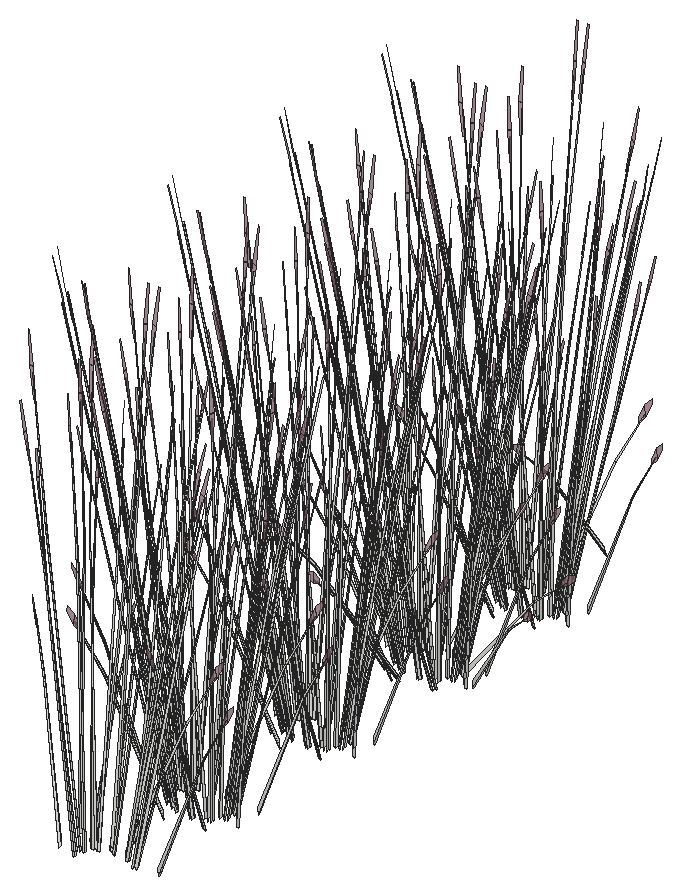
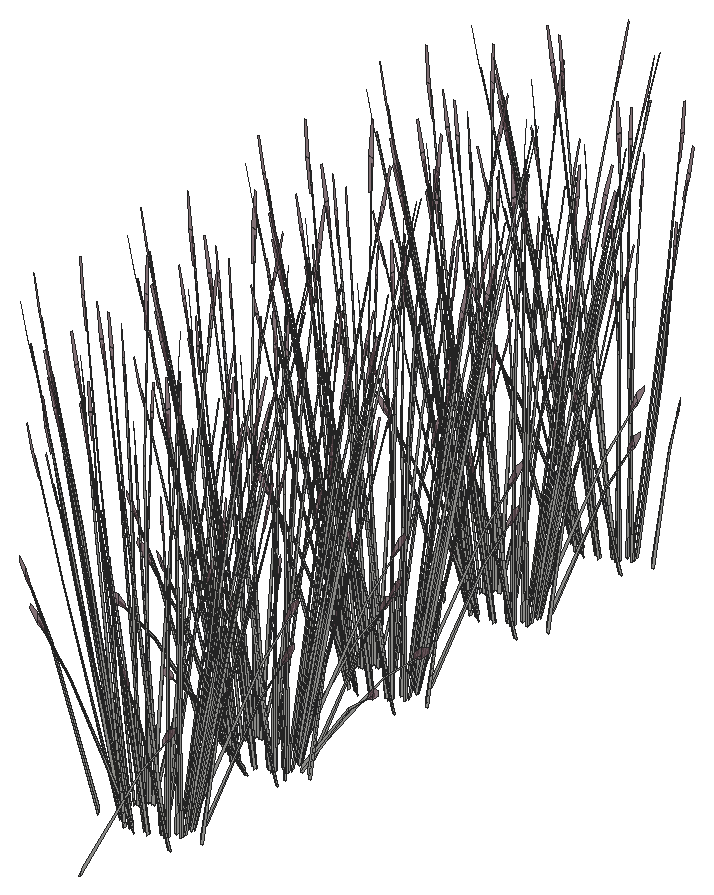
# SketchUp Ruby script. Lengths in inches.
U = 1.inch
M = Sketchup.active_model
def pt(a) = Geom::Point3d.new(a.map { |v| v * U })
def face(e, loops, mat)
  f = e.add_face(loops[0].map { |a| pt(a) })
  loops[1..].each { |l| e.add_face(l.map { |a| pt(a) }).erase! }
  f.material = f.back_material = mat if mat
  f
end
# faces: each face lists its corners as indices into pts; further lists are holes
def faces(e, pts, list, mat = nil) = list.each { |f| face(e, (f[0].is_a?(Array) ? f : [f]).map { |l| l.map { |i| pts[i] } }, mat) }
# xy, xz, yz: faces in a plane at the given z, y or x. An outline is a flat list of corners, or four numbers for a rectangle; further outlines are holes
def ring(l) = l.size == 4 ? [[l[0], l[1]], [l[2], l[1]], [l[2], l[3]], [l[0], l[3]]] : l.each_slice(2).to_a
def flat(e, list, mat, &to3) = list.each { |f| face(e, (f[0].is_a?(Array) ? f : [f]).map { |l| ring(l).map { |u, v| to3.(u, v) } }, mat) }
def xy(e, z, list, mat = nil) = flat(e, list, mat) { |x, y| [x, y, z] }
def xz(e, y, list, mat = nil) = flat(e, list, mat) { |x, z| [x, y, z] }
def yz(e, x, list, mat = nil) = flat(e, list, mat) { |y, z| [x, y, z] }
def lines(e, pts, list) = list.each { |a, b| e.add_line(pt(pts[a]), pt(pts[b])) }
# prism: a flat outline (further loops are holes) pulled along v
def prism(e, loops, v, mat = nil)
  f = face(e, loops, mat); d = Geom::Vector3d.new(v.map { |x| x * U })
  f.pushpull(f.normal.samedirection?(d) ? d.length : -d.length)
end
def box(e, o, s, mat = nil) = prism(e, [[o, [o[0] + s[0], o[1], o[2]], [o[0] + s[0], o[1] + s[1], o[2]], [o[0], o[1] + s[1], o[2]]]], [0, 0, s[2]], mat)
def at(x, y, z, deg = 0) = Geom::Transformation.translation(pt([x, y, z])) * Geom::Transformation.rotation(ORIGIN, Z_AXIS, deg.degrees)
def axes(o, x, y, z) = Geom::Transformation.new([*x, 0, *y, 0, *z, 0, *pt(o).to_a, 1])
def part(name) = M.definitions.add(name)
# library, detail: a bought-in or finely detailed component or shape, given as its bounding box
def library(name, o, s) = part(name).tap { |d| box(d.entities, o, s) }
def detail(e, o, s) = box(e.add_group.entities, o, s)
def put(e, d, t, mat = nil) = e.add_instance(d, t).tap { |i| i.material = mat if mat }
def group(e, t, mat = nil) = e.add_group.tap { |g| g.transformation = t; g.material = mat if mat }.entities
root = M.entities
M.materials.add("LightPink_Translucent").color = [144, 107, 117]
M.materials["LightPink_Translucent"].alpha = 0.75
c1 = part("blade")
p = [[2.15,0.21,22],[0,0.17,0],[0.09,0.45,0],[2.18,0.31,22],[2.29,0.31,22],[0.38,0.45,0],
  [2.48,0.24,33],[2.49,0.24,33],[2.48,0.22,33]]
faces(c1.entities,p,[[0,1,2,3],[4,5,2,3],[6,3,4,7],[8,0,3,6]])
c2 = part("seeds")
p = [[0.3,-0.1,1.38],[-0.01,-0.03,1.59],[-0.01,-0.03,0.03],[0.14,-0.07,-0.07],[0.29,-0.03,3],[0.15,0.01,3.11]]
faces(c2.entities,p,[[0,1,2,3],[1,0,4,5]],"LightPink_Translucent")
c3 = part("blade with seeds")
put(c3.entities,c1,at(0,0,0))
put(c3.entities,c2,axes([2.4,0.25,30.99],[1.5799,-0.05474,1.17369],[-0.12525,1.92788,0.29478],[-0.07173,-0.02425,1.56792]))
put(root,c3,axes([331.78,295.22,52.46],[0.41962,0.10901,0.31292],[-0.12239,0.31802,-0.40398],[-0.16894,0.02916,0.77298]))
put(root,c3,axes([337.02,296.95,52.16],[-0.04566,-0.03421,1.56736],[0.09987,-0.36669,-0.1481],[0.17984,-0.02343,0.27737]))
put(root,c3,axes([335.36,296.48,52.46],[-0.28729,-0.24465,0.31292],[0.32804,-0.23159,-0.40398],[0.16667,0.03524,0.77298]))
put(root,c3,axes([331.55,296.1,52.18],[-0.12522,-0.35963,0.42415],[0.49122,-0.06241,0.34973],[-0.14477,0.08458,0.87768]))
put(root,c3,axes([331.45,296.03,52.18],[-0.34663,-0.16434,0.05682],[0.20181,-0.23402,0.44729],[-0.11113,0.07566,0.68204]))
put(root,c3,axes([331.85,295.98,52.46],[0.43951,-0.05584,0.31292],[0.11606,0.31924,-0.40398],[-0.12595,0.08575,0.77298]))
put(root,c3,axes([330.16,295.84,52.16],[0.06444,0.01048,1.56736],[0.19934,0.34525,-0.1481],[-0.13191,0.09062,0.27737]))
put(root,c3,axes([335.62,296.7,52.18],[-0.02542,0.29714,0.05682],[-0.38391,-0.00815,0.44729],[0.14706,0.03109,0.68204]))
put(root,c3,axes([335.65,296.61,52.18],[-0.3723,0.25748,0.42415],[-0.32109,-0.27343,0.34973],[0.17467,0.04749,0.87768]))
put(root,c3,axes([330.85,296.89,52.99],[0.44556,0.1043,-0.05733],[-0.13706,0.32103,-0.25992],[-0.07288,0.04874,0.85731]))
put(root,c3,axes([334.47,296.9,52.46],[-0.07798,-0.31474,0.31292],[0.44579,-0.08311,-0.40398],[0.11974,0.09019,0.77298]))
put(root,c3,axes([332.45,296.62,52.46],[0.34164,-0.20573,0.31292],[0.3234,0.23491,-0.40398],[-0.04921,0.11936,0.77298]))
put(root,c3,axes([334.04,297.35,52.16],[0.00149,-0.04731,1.56736],[0.4327,-0.20872,-0.1481],[0.1503,0.0745,0.27737]))
put(root,c3,axes([332.14,296.8,52.18],[-0.41493,-0.01821,0.05682],[0.01138,-0.27493,0.44729],[-0.04342,0.10531,0.68204]))
put(root,c3,axes([332.27,296.83,52.18],[-0.35954,-0.26661,0.42415],[0.38183,-0.22994,0.34973],[-0.06632,0.12508,0.87768]))
put(root,c3,axes([333.4,296.95,52.46],[0.15222,-0.30049,0.31292],[0.44409,0.08764,-0.40398],[0.04072,0.12098,0.77298]))
put(root,c3,axes([334.54,297.19,52.18],[-0.22948,0.24822,0.05682],[-0.32679,-0.14452,0.44729],[0.10565,0.07958,0.68204]))
put(root,c3,axes([334,298.03,52.99],[0.34892,-0.22417,-0.05733],[0.3197,0.24551,-0.25992],[0.02251,0.06957,0.85731]))
put(root,c3,axes([334.64,297.12,52.18],[-0.5022,0.08967,0.42415],[-0.08716,-0.35177,0.34973],[0.11811,0.10367,0.87768]))
put(root,c3,axes([333.27,297.23,52.18],[-0.37205,0.1328,0.05682],[-0.18211,-0.24217,0.44729],[0.03593,0.10675,0.68204]))
put(root,c3,axes([332.23,296.67,52.77],[0.55492,0.01936,-0.11927],[-0.01517,0.36657,-0.66198],[-0.03855,0.14118,1.00587]))
put(root,c3,axes([333.4,297.2,52.47],[-0.49753,-0.10215,0.47081],[0.17013,-0.33585,0.3882],[0.0299,0.13207,0.97422]))
put(root,c3,axes([331.05,297.64,52.16],[0.05728,-0.02359,1.56736],[0.47345,0.15692,-0.1481],[-0.01113,0.13066,0.27737]))
put(root,c3,axes([335.78,302.96,52.16],[-0.05128,0.02985,1.56736],[-0.5024,-0.1007,-0.1481],[-0.01819,-0.13025,0.27737]))
put(root,c3,axes([333.05,302.39,52.16],[-0.00942,0.04684,1.56736],[-0.46458,0.16998,-0.1481],[-0.13671,-0.08689,0.27737]))
put(root,c3,axes([332.94,303.22,52.5],[0.56246,-0.10044,0.47505],[0.09762,0.39398,0.3917],[-0.13228,-0.11611,0.983]))
put(root,c3,axes([334.22,303.29,52.18],[0.49753,0.10215,0.42415],[-0.17013,0.33585,0.34973],[-0.0299,-0.13207,0.87768]))
put(root,c3,axes([334.35,303.27,52.18],[0.37205,-0.1328,0.05682],[0.18211,0.24217,0.44729],[-0.03593,-0.10675,0.68204]))
put(root,c3,axes([333.07,303.31,52.18],[0.22948,-0.24822,0.05682],[0.32679,0.14452,0.44729],[-0.10565,-0.07958,0.68204]))
put(root,c3,axes([334.21,303.54,52.46],[-0.15222,0.30049,0.31292],[-0.44409,-0.08764,-0.40398],[-0.04072,-0.12098,0.77298]))
put(root,c3,axes([335.34,303.67,52.18],[0.35954,0.26661,0.42415],[-0.38183,0.22994,0.34973],[0.06632,-0.12508,0.87768]))
put(root,c3,axes([333.18,303.28,52.8],[-0.33698,0.3746,-0.12034],[-0.48801,-0.21581,-0.66795],[-0.16964,-0.10584,1.01494]))
put(root,c3,axes([335.48,303.69,52.18],[0.41493,0.01821,0.05682],[-0.01138,0.27493,0.44729],[0.04342,-0.10531,0.68204]))
put(root,c3,axes([335.17,303.88,52.46],[-0.34164,0.20573,0.31292],[-0.3234,-0.23491,-0.40398],[0.04921,-0.11936,0.77298]))
put(root,c3,axes([333.14,303.59,52.46],[0.07798,0.31474,0.31292],[-0.44579,0.08311,-0.40398],[-0.11974,-0.09019,0.77298]))
put(root,c3,axes([331.8,303.8,52.5],[0.41698,-0.28837,0.47505],[0.35962,0.30624,0.3917],[-0.19563,-0.05319,0.983]))
put(root,c3,axes([337.14,304.45,52.16],[-0.06595,-0.00297,1.56736],[-0.27386,-0.31799,-0.1481],[0.10998,-0.10455,0.27737]))
put(root,c3,axes([331.99,303.79,52.18],[0.02542,-0.29714,0.05682],[0.38391,0.00815,0.44729],[-0.14706,-0.03109,0.68204]))
put(root,c3,axes([335.76,304.51,52.46],[-0.43951,0.05584,0.31292],[-0.11606,-0.31924,-0.40398],[0.12595,-0.08575,0.77298]))
put(root,c3,axes([336.16,304.46,52.18],[0.34663,0.16434,0.05682],[-0.20181,0.23402,0.44729],[0.11113,-0.07566,0.68204]))
put(root,c3,axes([336.0625,304.4,52.18],[0.12522,0.35963,0.42415],[-0.49122,0.06241,0.34973],[0.14477,-0.08458,0.87768]))
put(root,c3,axes([331.47,303.41,52.16],[0.03743,0.039,1.56736],[-0.18045,0.35054,-0.1481],[-0.18276,0.00254,0.27737]))
put(root,c3,axes([332.25,304.02,52.46],[0.28729,0.24465,0.31292],[-0.32804,0.23159,-0.40398],[-0.16667,-0.03524,0.77298]))
put(root,c3,axes([335.83,305.28,52.46],[-0.41962,-0.10901,0.31292],[0.12239,-0.31802,-0.40398],[0.16894,-0.02916,0.77298]))
put(root,c3,axes([331.4375,304.7,52.18],[0.14265,-0.35629,0.42415],[0.46898,0.12183,0.34973],[-0.18443,0.02141,0.87768]))
put(root,c3,axes([331.4,304.6,52.18],[-0.18545,-0.26643,0.05682],[0.33817,-0.13041,0.44729],[-0.14907,0.02573,0.68204]))
put(root,c3,axes([336.21,305.38,52.18],[0.18545,0.26643,0.05682],[-0.33817,0.13041,0.44729],[0.14907,-0.02573,0.68204]))
put(root,c3,axes([336.18,305.28,52.18],[-0.14265,0.35629,0.42415],[-0.46898,-0.12183,0.34973],[0.18443,-0.02141,0.87768]))
put(root,c3,axes([331.78,304.7,52.46],[0.41962,0.10901,0.31292],[-0.12239,0.31802,-0.40398],[-0.16894,0.02916,0.77298]))
put(root,c3,axes([337.02,306.4375,52.16],[-0.04566,-0.03421,1.56736],[0.09987,-0.36669,-0.1481],[0.17984,-0.02343,0.27737]))
put(root,c3,axes([335.36,305.96,52.46],[-0.28729,-0.24465,0.31292],[0.32804,-0.23159,-0.40398],[0.16667,0.03524,0.77298]))
put(root,c3,axes([331.55,305.58,52.18],[-0.12522,-0.35963,0.42415],[0.49122,-0.06241,0.34973],[-0.14477,0.08458,0.87768]))
put(root,c3,axes([331.45,305.52,52.18],[-0.34663,-0.16434,0.05682],[0.20181,-0.23402,0.44729],[-0.11113,0.07566,0.68204]))
put(root,c3,axes([331.85,305.46,52.46],[0.43951,-0.05584,0.31292],[0.11606,0.31924,-0.40398],[-0.12595,0.08575,0.77298]))
put(root,c3,axes([330.16,305.32,52.16],[0.06444,0.01048,1.56736],[0.19934,0.34525,-0.1481],[-0.13191,0.09062,0.27737]))
put(root,c3,axes([335.62,306.1875,52.18],[-0.02542,0.29714,0.05682],[-0.38391,-0.00815,0.44729],[0.14706,0.03109,0.68204]))
put(root,c3,axes([335.65,306.09,52.18],[-0.3723,0.25748,0.42415],[-0.32109,-0.27343,0.34973],[0.17467,0.04749,0.87768]))
put(root,c3,axes([330.85,306.37,52.99],[0.44556,0.1043,-0.05733],[-0.13706,0.32103,-0.25992],[-0.07288,0.04874,0.85731]))
put(root,c3,axes([334.47,306.39,52.46],[-0.07798,-0.31474,0.31292],[0.44579,-0.08311,-0.40398],[0.11974,0.09019,0.77298]))
put(root,c3,axes([332.45,306.1,52.46],[0.34164,-0.20573,0.31292],[0.3234,0.23491,-0.40398],[-0.04921,0.11936,0.77298]))
put(root,c3,axes([334.04,306.83,52.16],[0.00149,-0.04731,1.56736],[0.4327,-0.20872,-0.1481],[0.1503,0.0745,0.27737]))
put(root,c3,axes([332.14,306.29,52.18],[-0.41493,-0.01821,0.05682],[0.01138,-0.27493,0.44729],[-0.04342,0.10531,0.68204]))
put(root,c3,axes([332.27,306.3125,52.18],[-0.35954,-0.26661,0.42415],[0.38183,-0.22994,0.34973],[-0.06632,0.12508,0.87768]))
put(root,c3,axes([333.4,306.4375,52.46],[0.15222,-0.30049,0.31292],[0.44409,0.08764,-0.40398],[0.04072,0.12098,0.77298]))
put(root,c3,axes([334.54,306.67,52.18],[-0.22948,0.24822,0.05682],[-0.32679,-0.14452,0.44729],[0.10565,0.07958,0.68204]))
put(root,c3,axes([334,307.51,52.99],[0.34892,-0.22417,-0.05733],[0.3197,0.24551,-0.25992],[0.02251,0.06957,0.85731]))
put(root,c3,axes([334.64,306.61,52.18],[-0.5022,0.08967,0.42415],[-0.08716,-0.35177,0.34973],[0.11811,0.10367,0.87768]))
put(root,c3,axes([333.27,306.71,52.18],[-0.37205,0.1328,0.05682],[-0.18211,-0.24217,0.44729],[0.03593,0.10675,0.68204]))
put(root,c3,axes([332.23,306.16,52.77],[0.55492,0.01936,-0.11927],[-0.01517,0.36657,-0.66198],[-0.03855,0.14118,1.00587]))
put(root,c3,axes([333.4,306.6875,52.47],[-0.49753,-0.10215,0.47081],[0.17013,-0.33585,0.3882],[0.0299,0.13207,0.97422]))
put(root,c3,axes([331.05,307.125,52.16],[0.05728,-0.02359,1.56736],[0.47345,0.15692,-0.1481],[-0.01113,0.13066,0.27737]))
put(root,c3,axes([335.78,313.95,52.16],[-0.05128,0.02985,1.56736],[-0.5024,-0.1007,-0.1481],[-0.01819,-0.13025,0.27737]))
put(root,c3,axes([333.05,313.38,52.16],[-0.00942,0.04684,1.56736],[-0.46458,0.16998,-0.1481],[-0.13671,-0.08689,0.27737]))
put(root,c3,axes([332.94,314.21,52.5],[0.56246,-0.10044,0.47505],[0.09762,0.39398,0.3917],[-0.13228,-0.11611,0.983]))
put(root,c3,axes([334.22,314.28,52.18],[0.49753,0.10215,0.42415],[-0.17013,0.33585,0.34973],[-0.0299,-0.13207,0.87768]))
put(root,c3,axes([334.35,314.26,52.18],[0.37205,-0.1328,0.05682],[0.18211,0.24217,0.44729],[-0.03593,-0.10675,0.68204]))
put(root,c3,axes([333.07,314.29,52.18],[0.22948,-0.24822,0.05682],[0.32679,0.14452,0.44729],[-0.10565,-0.07958,0.68204]))
put(root,c3,axes([334.21,314.53,52.46],[-0.15222,0.30049,0.31292],[-0.44409,-0.08764,-0.40398],[-0.04072,-0.12098,0.77298]))
put(root,c3,axes([335.34,314.66,52.18],[0.35954,0.26661,0.42415],[-0.38183,0.22994,0.34973],[0.06632,-0.12508,0.87768]))
put(root,c3,axes([333.18,314.27,52.8],[-0.33698,0.3746,-0.12034],[-0.48801,-0.21581,-0.66795],[-0.16964,-0.10584,1.01494]))
put(root,c3,axes([335.48,314.68,52.18],[0.41493,0.01821,0.05682],[-0.01138,0.27493,0.44729],[0.04342,-0.10531,0.68204]))
put(root,c3,axes([335.17,314.87,52.46],[-0.34164,0.20573,0.31292],[-0.3234,-0.23491,-0.40398],[0.04921,-0.11936,0.77298]))
put(root,c3,axes([333.14,314.58,52.46],[0.07798,0.31474,0.31292],[-0.44579,0.08311,-0.40398],[-0.11974,-0.09019,0.77298]))
put(root,c3,axes([331.8,314.78,52.5],[0.41698,-0.28837,0.47505],[0.35962,0.30624,0.3917],[-0.19563,-0.05319,0.983]))
put(root,c3,axes([337.14,315.4375,52.16],[-0.06595,-0.00297,1.56736],[-0.27386,-0.31799,-0.1481],[0.10998,-0.10455,0.27737]))
put(root,c3,axes([331.99,314.78,52.18],[0.02542,-0.29714,0.05682],[0.38391,0.00815,0.44729],[-0.14706,-0.03109,0.68204]))
put(root,c3,axes([335.76,315.5,52.46],[-0.43951,0.05584,0.31292],[-0.11606,-0.31924,-0.40398],[0.12595,-0.08575,0.77298]))
put(root,c3,axes([336.16,315.45,52.18],[0.34663,0.16434,0.05682],[-0.20181,0.23402,0.44729],[0.11113,-0.07566,0.68204]))
put(root,c3,axes([336.0625,315.38,52.18],[0.12522,0.35963,0.42415],[-0.49122,0.06241,0.34973],[0.14477,-0.08458,0.87768]))
put(root,c3,axes([331.47,314.39,52.16],[0.03743,0.039,1.56736],[-0.18045,0.35054,-0.1481],[-0.18276,0.00254,0.27737]))
put(root,c3,axes([332.25,315,52.46],[0.28729,0.24465,0.31292],[-0.32804,0.23159,-0.40398],[-0.16667,-0.03524,0.77298]))
put(root,c3,axes([335.83,316.27,52.46],[-0.41962,-0.10901,0.31292],[0.12239,-0.31802,-0.40398],[0.16894,-0.02916,0.77298]))
put(root,c3,axes([331.4375,315.6875,52.18],[0.14265,-0.35629,0.42415],[0.46898,0.12183,0.34973],[-0.18443,0.02141,0.87768]))
put(root,c3,axes([331.4,315.59,52.18],[-0.18545,-0.26643,0.05682],[0.33817,-0.13041,0.44729],[-0.14907,0.02573,0.68204]))
put(root,c3,axes([336.21,316.37,52.18],[0.18545,0.26643,0.05682],[-0.33817,0.13041,0.44729],[0.14907,-0.02573,0.68204]))
put(root,c3,axes([336.18,316.27,52.18],[-0.14265,0.35629,0.42415],[-0.46898,-0.12183,0.34973],[0.18443,-0.02141,0.87768]))
put(root,c3,axes([331.78,315.69,52.46],[0.41962,0.10901,0.31292],[-0.12239,0.31802,-0.40398],[-0.16894,0.02916,0.77298]))
put(root,c3,axes([337.02,317.42,52.16],[-0.04566,-0.03421,1.56736],[0.09987,-0.36669,-0.1481],[0.17984,-0.02343,0.27737]))
put(root,c3,axes([335.36,316.95,52.46],[-0.28729,-0.24465,0.31292],[0.32804,-0.23159,-0.40398],[0.16667,0.03524,0.77298]))
put(root,c3,axes([331.55,316.57,52.18],[-0.12522,-0.35963,0.42415],[0.49122,-0.06241,0.34973],[-0.14477,0.08458,0.87768]))
put(root,c3,axes([331.45,316.5,52.18],[-0.34663,-0.16434,0.05682],[0.20181,-0.23402,0.44729],[-0.11113,0.07566,0.68204]))
put(root,c3,axes([331.85,316.45,52.46],[0.43951,-0.05584,0.31292],[0.11606,0.31924,-0.40398],[-0.12595,0.08575,0.77298]))
put(root,c3,axes([330.16,316.3125,52.16],[0.06444,0.01048,1.56736],[0.19934,0.34525,-0.1481],[-0.13191,0.09062,0.27737]))
put(root,c3,axes([335.62,317.18,52.18],[-0.02542,0.29714,0.05682],[-0.38391,-0.00815,0.44729],[0.14706,0.03109,0.68204]))
put(root,c3,axes([335.65,317.08,52.18],[-0.3723,0.25748,0.42415],[-0.32109,-0.27343,0.34973],[0.17467,0.04749,0.87768]))
put(root,c3,axes([330.85,317.36,52.99],[0.44556,0.1043,-0.05733],[-0.13706,0.32103,-0.25992],[-0.07288,0.04874,0.85731]))
put(root,c3,axes([334.47,317.38,52.46],[-0.07798,-0.31474,0.31292],[0.44579,-0.08311,-0.40398],[0.11974,0.09019,0.77298]))
put(root,c3,axes([332.45,317.09,52.46],[0.34164,-0.20573,0.31292],[0.3234,0.23491,-0.40398],[-0.04921,0.11936,0.77298]))
put(root,c3,axes([334.04,317.82,52.16],[0.00149,-0.04731,1.56736],[0.4327,-0.20872,-0.1481],[0.1503,0.0745,0.27737]))
put(root,c3,axes([332.14,317.28,52.18],[-0.41493,-0.01821,0.05682],[0.01138,-0.27493,0.44729],[-0.04342,0.10531,0.68204]))
put(root,c3,axes([332.27,317.3,52.18],[-0.35954,-0.26661,0.42415],[0.38183,-0.22994,0.34973],[-0.06632,0.12508,0.87768]))
put(root,c3,axes([333.4,317.43,52.46],[0.15222,-0.30049,0.31292],[0.44409,0.08764,-0.40398],[0.04072,0.12098,0.77298]))
put(root,c3,axes([334.54,317.66,52.18],[-0.22948,0.24822,0.05682],[-0.32679,-0.14452,0.44729],[0.10565,0.07958,0.68204]))
put(root,c3,axes([334,318.5,52.99],[0.34892,-0.22417,-0.05733],[0.3197,0.24551,-0.25992],[0.02251,0.06957,0.85731]))
put(root,c3,axes([334.64,317.59,52.18],[-0.5022,0.08967,0.42415],[-0.08716,-0.35177,0.34973],[0.11811,0.10367,0.87768]))
put(root,c3,axes([333.27,317.7,52.18],[-0.37205,0.1328,0.05682],[-0.18211,-0.24217,0.44729],[0.03593,0.10675,0.68204]))
put(root,c3,axes([332.23,317.15,52.77],[0.55492,0.01936,-0.11927],[-0.01517,0.36657,-0.66198],[-0.03855,0.14118,1.00587]))
put(root,c3,axes([333.4,317.68,52.47],[-0.49753,-0.10215,0.47081],[0.17013,-0.33585,0.3882],[0.0299,0.13207,0.97422]))
put(root,c3,axes([331.05,318.11,52.16],[0.05728,-0.02359,1.56736],[0.47345,0.15692,-0.1481],[-0.01113,0.13066,0.27737]))
put(root,c3,axes([333.57,324.16,52.17],[-0.07723,-0.05479,1.54581],[-0.51538,0.03473,-0.24447],[-0.08225,-0.13104,0.12397]))
put(root,c3,axes([335.89,324.83,52.17],[-0.00487,-0.07777,1.54581],[-0.41166,-0.22476,-0.24447],[0.06364,-0.13625,0.12397]))
put(root,c3,axes([335.78,324.55,52.16],[-0.05128,0.02985,1.56736],[-0.5024,-0.1007,-0.1481],[-0.01819,-0.13025,0.27737]))
put(root,c3,axes([333.05,323.98,52.16],[-0.00942,0.04684,1.56736],[-0.46458,0.16998,-0.1481],[-0.13671,-0.08689,0.27737]))
put(root,c3,axes([332.94,324.81,52.5],[0.56246,-0.10044,0.47505],[0.09762,0.39398,0.3917],[-0.13228,-0.11611,0.983]))
put(root,c3,axes([334.22,324.88,52.18],[0.49753,0.10215,0.42415],[-0.17013,0.33585,0.34973],[-0.0299,-0.13207,0.87768]))
put(root,c3,axes([334.35,324.85,52.18],[0.37205,-0.1328,0.05682],[0.18211,0.24217,0.44729],[-0.03593,-0.10675,0.68204]))
put(root,c3,axes([333.07,324.89,52.18],[0.22948,-0.24822,0.05682],[0.32679,0.14452,0.44729],[-0.10565,-0.07958,0.68204]))
put(root,c3,axes([334.21,325.13,52.46],[-0.15222,0.30049,0.31292],[-0.44409,-0.08764,-0.40398],[-0.04072,-0.12098,0.77298]))
put(root,c3,axes([335.34,325.25,52.18],[0.35954,0.26661,0.42415],[-0.38183,0.22994,0.34973],[0.06632,-0.12508,0.87768]))
put(root,c3,axes([333.18,324.87,52.8],[-0.33698,0.3746,-0.12034],[-0.48801,-0.21581,-0.66795],[-0.16964,-0.10584,1.01494]))
put(root,c3,axes([335.48,325.28,52.18],[0.41493,0.01821,0.05682],[-0.01138,0.27493,0.44729],[0.04342,-0.10531,0.68204]))
put(root,c3,axes([335.17,325.47,52.46],[-0.34164,0.20573,0.31292],[-0.3234,-0.23491,-0.40398],[0.04921,-0.11936,0.77298]))
put(root,c3,axes([331.88,324.76,52.17],[-0.10864,-0.00276,1.54581],[-0.34587,0.27582,-0.24447],[-0.18454,-0.05636,0.12397]))
put(root,c3,axes([333.14,325.18,52.46],[0.07798,0.31474,0.31292],[-0.44579,0.08311,-0.40398],[-0.11974,-0.09019,0.77298]))
put(root,c3,axes([331.8,325.38,52.5],[0.41698,-0.28837,0.47505],[0.35962,0.30624,0.3917],[-0.19563,-0.05319,0.983]))
put(root,c3,axes([337.14,326.04,52.16],[-0.06595,-0.00297,1.56736],[-0.27386,-0.31799,-0.1481],[0.10998,-0.10455,0.27737]))
put(root,c3,axes([331.99,325.38,52.18],[0.02542,-0.29714,0.05682],[0.38391,0.00815,0.44729],[-0.14706,-0.03109,0.68204]))
put(root,c3,axes([335.76,326.1,52.46],[-0.43951,0.05584,0.31292],[-0.11606,-0.31924,-0.40398],[0.12595,-0.08575,0.77298]))
put(root,c3,axes([336.16,326.05,52.18],[0.34663,0.16434,0.05682],[-0.20181,0.23402,0.44729],[0.11113,-0.07566,0.68204]))
put(root,c3,axes([336.0625,325.98,52.18],[0.12522,0.35963,0.42415],[-0.49122,0.06241,0.34973],[0.14477,-0.08458,0.87768]))
put(root,c3,axes([337.39,326.42,52.17],[0.07006,-0.05952,1.54581],[-0.08968,-0.3651,-0.24447],[0.1758,-0.06922,0.12397]))
put(root,c3,axes([331.47,324.99,52.16],[0.03743,0.039,1.56736],[-0.18045,0.35054,-0.1481],[-0.18276,0.00254,0.27737]))
put(root,c3,axes([332.25,325.6,52.46],[0.28729,0.24465,0.31292],[-0.32804,0.23159,-0.40398],[-0.16667,-0.03524,0.77298]))
put(root,c3,axes([335.83,326.86,52.46],[-0.41962,-0.10901,0.31292],[0.12239,-0.31802,-0.40398],[0.16894,-0.02916,0.77298]))
put(root,c3,axes([331.4375,326.28,52.18],[0.14265,-0.35629,0.42415],[0.46898,0.12183,0.34973],[-0.18443,0.02141,0.87768]))
put(root,c3,axes([331.4,326.1875,52.18],[-0.18545,-0.26643,0.05682],[0.33817,-0.13041,0.44729],[-0.14907,0.02573,0.68204]))
put(root,c3,axes([336.21,326.96,52.18],[0.18545,0.26643,0.05682],[-0.33817,0.13041,0.44729],[0.14907,-0.02573,0.68204]))
put(root,c3,axes([336.18,326.87,52.18],[-0.14265,0.35629,0.42415],[-0.46898,-0.12183,0.34973],[0.18443,-0.02141,0.87768]))
put(root,c3,axes([331.78,326.29,52.46],[0.41962,0.10901,0.31292],[-0.12239,0.31802,-0.40398],[-0.16894,0.02916,0.77298]))
put(root,c3,axes([337.02,328.02,52.16],[-0.04566,-0.03421,1.56736],[0.09987,-0.36669,-0.1481],[0.17984,-0.02343,0.27737]))
put(root,c3,axes([331.08,326.53,52.17],[-0.08245,0.05073,1.54581],[0.00701,0.37067,-0.24447],[-0.18899,0.0482,0.12397]))
put(root,c3,axes([335.36,327.55,52.46],[-0.28729,-0.24465,0.31292],[0.32804,-0.23159,-0.40398],[0.16667,0.03524,0.77298]))
put(root,c3,axes([335.88,327.47,52.17],[0.10831,-0.00661,1.54581],[0.29709,-0.30358,-0.24447],[0.19266,0.04007,0.12397]))
put(root,c3,axes([331.55,327.17,52.18],[-0.12522,-0.35963,0.42415],[0.49122,-0.06241,0.34973],[-0.14477,0.08458,0.87768]))
put(root,c3,axes([331.45,327.1,52.18],[-0.34663,-0.16434,0.05682],[0.20181,-0.23402,0.44729],[-0.11113,0.07566,0.68204]))
put(root,c3,axes([331.85,327.05,52.46],[0.43951,-0.05584,0.31292],[0.11606,0.31924,-0.40398],[-0.12595,0.08575,0.77298]))
put(root,c3,axes([330.16,326.91,52.16],[0.06444,0.01048,1.56736],[0.19934,0.34525,-0.1481],[-0.13191,0.09062,0.27737]))
put(root,c3,axes([335.62,327.77,52.18],[-0.02542,0.29714,0.05682],[-0.38391,-0.00815,0.44729],[0.14706,0.03109,0.68204]))
put(root,c3,axes([335.65,327.68,52.18],[-0.3723,0.25748,0.42415],[-0.32109,-0.27343,0.34973],[0.17467,0.04749,0.87768]))
put(root,c3,axes([330.85,327.96,52.99],[0.44556,0.1043,-0.05733],[-0.13706,0.32103,-0.25992],[-0.07288,0.04874,0.85731]))
put(root,c3,axes([334.47,327.98,52.46],[-0.07798,-0.31474,0.31292],[0.44579,-0.08311,-0.40398],[0.11974,0.09019,0.77298]))
put(root,c3,axes([332.45,327.6875,52.46],[0.34164,-0.20573,0.31292],[0.3234,0.23491,-0.40398],[-0.04921,0.11936,0.77298]))
put(root,c3,axes([334.04,328.42,52.16],[0.00149,-0.04731,1.56736],[0.4327,-0.20872,-0.1481],[0.1503,0.0745,0.27737]))
put(root,c3,axes([332.14,327.875,52.18],[-0.41493,-0.01821,0.05682],[0.01138,-0.27493,0.44729],[-0.04342,0.10531,0.68204]))
put(root,c3,axes([332.27,327.9,52.18],[-0.35954,-0.26661,0.42415],[0.38183,-0.22994,0.34973],[-0.06632,0.12508,0.87768]))
put(root,c3,axes([333.4,328.03,52.46],[0.15222,-0.30049,0.31292],[0.44409,0.08764,-0.40398],[0.04072,0.12098,0.77298]))
put(root,c3,axes([334.54,328.26,52.18],[-0.22948,0.24822,0.05682],[-0.32679,-0.14452,0.44729],[0.10565,0.07958,0.68204]))
put(root,c3,axes([334,329.1,52.99],[0.34892,-0.22417,-0.05733],[0.3197,0.24551,-0.25992],[0.02251,0.06957,0.85731]))
put(root,c3,axes([334.64,328.19,52.18],[-0.5022,0.08967,0.42415],[-0.08716,-0.35177,0.34973],[0.11811,0.10367,0.87768]))
put(root,c3,axes([333.27,328.3,52.18],[-0.37205,0.1328,0.05682],[-0.18211,-0.24217,0.44729],[0.03593,0.10675,0.68204]))
put(root,c3,axes([331.09,327.92,52.17],[-0.01255,0.07733,1.54581],[0.35618,0.269,-0.24447],[-0.09325,0.12721,0.12397]))
put(root,c3,axes([332.23,327.74,52.77],[0.55492,0.01936,-0.11927],[-0.01517,0.36657,-0.66198],[-0.03855,0.14118,1.00587]))
put(root,c3,axes([333.4,328.27,52.47],[-0.49753,-0.10215,0.47081],[0.17013,-0.33585,0.3882],[0.0299,0.13207,0.97422]))
put(root,c3,axes([331.05,328.71,52.16],[0.05728,-0.02359,1.56736],[0.47345,0.15692,-0.1481],[-0.01113,0.13066,0.27737]))
put(root,c3,axes([333.14,328.875,52.17],[0.064,0.06292,1.54581],[0.51651,0.02472,-0.24447],[0.05194,0.13877,0.12397]))
put(root,c3,axes([335.78,334.25,52.16],[-0.05128,0.02985,1.56736],[-0.5024,-0.1007,-0.1481],[-0.01819,-0.13025,0.27737]))
put(root,c3,axes([333.05,333.68,52.16],[-0.00942,0.04684,1.56736],[-0.46458,0.16998,-0.1481],[-0.13671,-0.08689,0.27737]))
put(root,c3,axes([332.94,334.51,52.5],[0.56246,-0.10044,0.47505],[0.09762,0.39398,0.3917],[-0.13228,-0.11611,0.983]))
put(root,c3,axes([334.22,334.58,52.18],[0.49753,0.10215,0.42415],[-0.17013,0.33585,0.34973],[-0.0299,-0.13207,0.87768]))
put(root,c3,axes([334.35,334.56,52.18],[0.37205,-0.1328,0.05682],[0.18211,0.24217,0.44729],[-0.03593,-0.10675,0.68204]))
put(root,c3,axes([333.07,334.6,52.18],[0.22948,-0.24822,0.05682],[0.32679,0.14452,0.44729],[-0.10565,-0.07958,0.68204]))
put(root,c3,axes([334.21,334.83,52.46],[-0.15222,0.30049,0.31292],[-0.44409,-0.08764,-0.40398],[-0.04072,-0.12098,0.77298]))
put(root,c3,axes([335.34,334.96,52.18],[0.35954,0.26661,0.42415],[-0.38183,0.22994,0.34973],[0.06632,-0.12508,0.87768]))
put(root,c3,axes([333.18,334.57,52.8],[-0.33698,0.3746,-0.12034],[-0.48801,-0.21581,-0.66795],[-0.16964,-0.10584,1.01494]))
put(root,c3,axes([335.48,334.98,52.18],[0.41493,0.01821,0.05682],[-0.01138,0.27493,0.44729],[0.04342,-0.10531,0.68204]))
put(root,c3,axes([335.17,335.17,52.46],[-0.34164,0.20573,0.31292],[-0.3234,-0.23491,-0.40398],[0.04921,-0.11936,0.77298]))
put(root,c3,axes([333.14,334.88,52.46],[0.07798,0.31474,0.31292],[-0.44579,0.08311,-0.40398],[-0.11974,-0.09019,0.77298]))
put(root,c3,axes([331.8,335.09,52.5],[0.41698,-0.28837,0.47505],[0.35962,0.30624,0.3917],[-0.19563,-0.05319,0.983]))
put(root,c3,axes([337.14,335.74,52.16],[-0.06595,-0.00297,1.56736],[-0.27386,-0.31799,-0.1481],[0.10998,-0.10455,0.27737]))
put(root,c3,axes([331.99,335.08,52.18],[0.02542,-0.29714,0.05682],[0.38391,0.00815,0.44729],[-0.14706,-0.03109,0.68204]))
put(root,c3,axes([335.76,335.81,52.46],[-0.43951,0.05584,0.31292],[-0.11606,-0.31924,-0.40398],[0.12595,-0.08575,0.77298]))
put(root,c3,axes([336.16,335.76,52.18],[0.34663,0.16434,0.05682],[-0.20181,0.23402,0.44729],[0.11113,-0.07566,0.68204]))
put(root,c3,axes([336.0625,335.6875,52.18],[0.12522,0.35963,0.42415],[-0.49122,0.06241,0.34973],[0.14477,-0.08458,0.87768]))
put(root,c3,axes([331.47,334.7,52.16],[0.03743,0.039,1.56736],[-0.18045,0.35054,-0.1481],[-0.18276,0.00254,0.27737]))
put(root,c3,axes([332.25,335.31,52.46],[0.28729,0.24465,0.31292],[-0.32804,0.23159,-0.40398],[-0.16667,-0.03524,0.77298]))
put(root,c3,axes([335.83,336.57,52.46],[-0.41962,-0.10901,0.31292],[0.12239,-0.31802,-0.40398],[0.16894,-0.02916,0.77298]))
put(root,c3,axes([331.4375,335.99,52.18],[0.14265,-0.35629,0.42415],[0.46898,0.12183,0.34973],[-0.18443,0.02141,0.87768]))
put(root,c3,axes([331.4,335.89,52.18],[-0.18545,-0.26643,0.05682],[0.33817,-0.13041,0.44729],[-0.14907,0.02573,0.68204]))
put(root,c3,axes([336.21,336.67,52.18],[0.18545,0.26643,0.05682],[-0.33817,0.13041,0.44729],[0.14907,-0.02573,0.68204]))
put(root,c3,axes([336.18,336.57,52.18],[-0.14265,0.35629,0.42415],[-0.46898,-0.12183,0.34973],[0.18443,-0.02141,0.87768]))
put(root,c3,axes([331.78,335.99,52.46],[0.41962,0.10901,0.31292],[-0.12239,0.31802,-0.40398],[-0.16894,0.02916,0.77298]))
put(root,c3,axes([337.02,337.73,52.16],[-0.04566,-0.03421,1.56736],[0.09987,-0.36669,-0.1481],[0.17984,-0.02343,0.27737]))
put(root,c3,axes([335.36,337.26,52.46],[-0.28729,-0.24465,0.31292],[0.32804,-0.23159,-0.40398],[0.16667,0.03524,0.77298]))
put(root,c3,axes([331.55,336.875,52.18],[-0.12522,-0.35963,0.42415],[0.49122,-0.06241,0.34973],[-0.14477,0.08458,0.87768]))
put(root,c3,axes([331.45,336.81,52.18],[-0.34663,-0.16434,0.05682],[0.20181,-0.23402,0.44729],[-0.11113,0.07566,0.68204]))
put(root,c3,axes([331.85,336.76,52.46],[0.43951,-0.05584,0.31292],[0.11606,0.31924,-0.40398],[-0.12595,0.08575,0.77298]))
put(root,c3,axes([330.16,336.61,52.16],[0.06444,0.01048,1.56736],[0.19934,0.34525,-0.1481],[-0.13191,0.09062,0.27737]))
put(root,c3,axes([335.62,337.48,52.18],[-0.02542,0.29714,0.05682],[-0.38391,-0.00815,0.44729],[0.14706,0.03109,0.68204]))
put(root,c3,axes([335.65,337.38,52.18],[-0.3723,0.25748,0.42415],[-0.32109,-0.27343,0.34973],[0.17467,0.04749,0.87768]))
put(root,c3,axes([330.85,337.66,52.99],[0.44556,0.1043,-0.05733],[-0.13706,0.32103,-0.25992],[-0.07288,0.04874,0.85731]))
put(root,c3,axes([334.47,337.68,52.46],[-0.07798,-0.31474,0.31292],[0.44579,-0.08311,-0.40398],[0.11974,0.09019,0.77298]))
put(root,c3,axes([332.45,337.39,52.46],[0.34164,-0.20573,0.31292],[0.3234,0.23491,-0.40398],[-0.04921,0.11936,0.77298]))
put(root,c3,axes([334.04,338.12,52.16],[0.00149,-0.04731,1.56736],[0.4327,-0.20872,-0.1481],[0.1503,0.0745,0.27737]))
put(root,c3,axes([332.14,337.58,52.18],[-0.41493,-0.01821,0.05682],[0.01138,-0.27493,0.44729],[-0.04342,0.10531,0.68204]))
put(root,c3,axes([332.27,337.6,52.18],[-0.35954,-0.26661,0.42415],[0.38183,-0.22994,0.34973],[-0.06632,0.12508,0.87768]))
put(root,c3,axes([333.4,337.73,52.46],[0.15222,-0.30049,0.31292],[0.44409,0.08764,-0.40398],[0.04072,0.12098,0.77298]))
put(root,c3,axes([334.54,337.97,52.18],[-0.22948,0.24822,0.05682],[-0.32679,-0.14452,0.44729],[0.10565,0.07958,0.68204]))
put(root,c3,axes([334,338.8,52.99],[0.34892,-0.22417,-0.05733],[0.3197,0.24551,-0.25992],[0.02251,0.06957,0.85731]))
put(root,c3,axes([334.64,337.9,52.18],[-0.5022,0.08967,0.42415],[-0.08716,-0.35177,0.34973],[0.11811,0.10367,0.87768]))
put(root,c3,axes([333.27,338,52.18],[-0.37205,0.1328,0.05682],[-0.18211,-0.24217,0.44729],[0.03593,0.10675,0.68204]))
put(root,c3,axes([332.23,337.45,52.77],[0.55492,0.01936,-0.11927],[-0.01517,0.36657,-0.66198],[-0.03855,0.14118,1.00587]))
put(root,c3,axes([333.4,337.98,52.47],[-0.49753,-0.10215,0.47081],[0.17013,-0.33585,0.3882],[0.0299,0.13207,0.97422]))
put(root,c3,axes([331.05,338.42,52.16],[0.05728,-0.02359,1.56736],[0.47345,0.15692,-0.1481],[-0.01113,0.13066,0.27737]))
put(root,c3,axes([333.57,343.79,52.17],[-0.07723,-0.05479,1.54581],[-0.51538,0.03473,-0.24447],[-0.08225,-0.13104,0.12397]))
